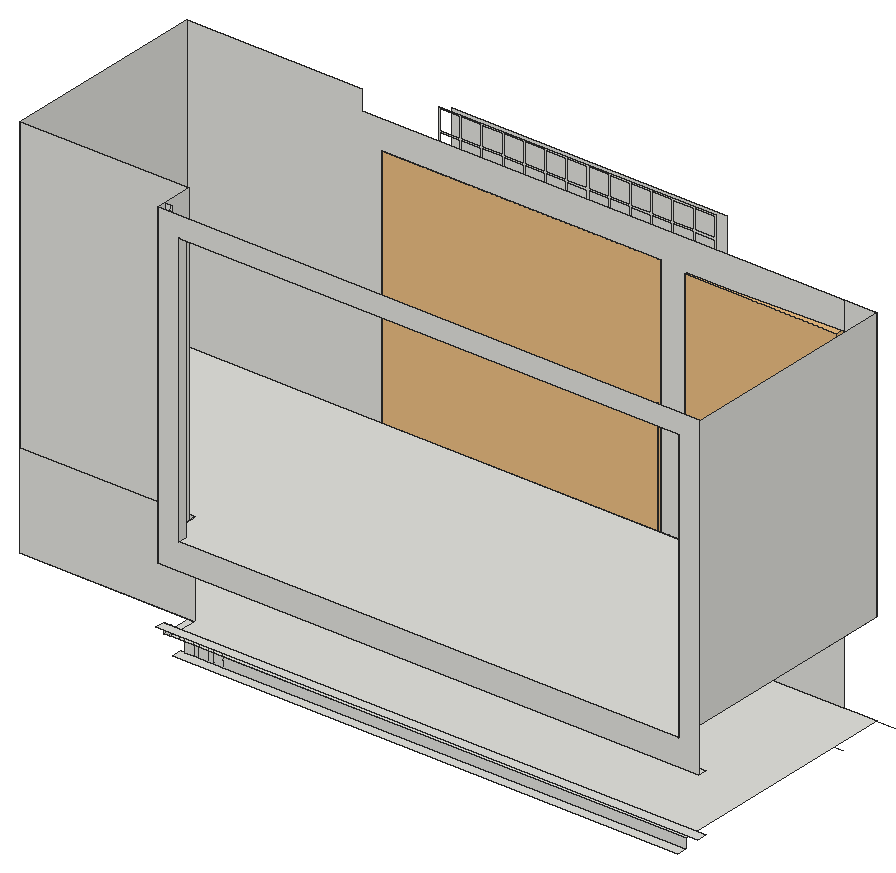
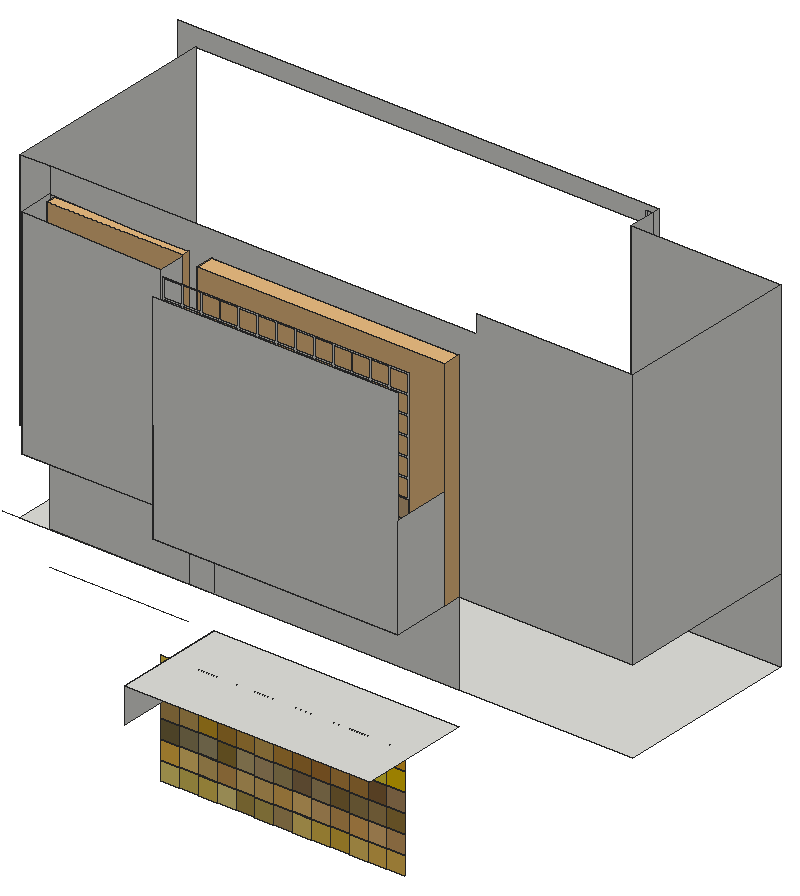
# SketchUp Ruby script. Lengths in inches.
U = 1.inch
M = Sketchup.active_model
def pt(a) = Geom::Point3d.new(a.map { |v| v * U })
def face(e, loops, mat)
  f = e.add_face(loops[0].map { |a| pt(a) })
  loops[1..].each { |l| e.add_face(l.map { |a| pt(a) }).erase! }
  f.material = f.back_material = mat if mat
  f
end
# faces: each face lists its corners as indices into pts; further lists are holes
def faces(e, pts, list, mat = nil) = list.each { |f| face(e, (f[0].is_a?(Array) ? f : [f]).map { |l| l.map { |i| pts[i] } }, mat) }
# xy, xz, yz: faces in a plane at the given z, y or x. An outline is a flat list of corners, or four numbers for a rectangle; further outlines are holes
def ring(l) = l.size == 4 ? [[l[0], l[1]], [l[2], l[1]], [l[2], l[3]], [l[0], l[3]]] : l.each_slice(2).to_a
def flat(e, list, mat, &to3) = list.each { |f| face(e, (f[0].is_a?(Array) ? f : [f]).map { |l| ring(l).map { |u, v| to3.(u, v) } }, mat) }
def xy(e, z, list, mat = nil) = flat(e, list, mat) { |x, y| [x, y, z] }
def xz(e, y, list, mat = nil) = flat(e, list, mat) { |x, z| [x, y, z] }
def yz(e, x, list, mat = nil) = flat(e, list, mat) { |y, z| [x, y, z] }
def lines(e, pts, list) = list.each { |a, b| e.add_line(pt(pts[a]), pt(pts[b])) }
# prism: a flat outline (further loops are holes) pulled along v
def prism(e, loops, v, mat = nil)
  f = face(e, loops, mat); d = Geom::Vector3d.new(v.map { |x| x * U })
  f.pushpull(f.normal.samedirection?(d) ? d.length : -d.length)
end
def box(e, o, s, mat = nil) = prism(e, [[o, [o[0] + s[0], o[1], o[2]], [o[0] + s[0], o[1] + s[1], o[2]], [o[0], o[1] + s[1], o[2]]]], [0, 0, s[2]], mat)
def at(x, y, z, deg = 0) = Geom::Transformation.translation(pt([x, y, z])) * Geom::Transformation.rotation(ORIGIN, Z_AXIS, deg.degrees)
def axes(o, x, y, z) = Geom::Transformation.new([*x, 0, *y, 0, *z, 0, *pt(o).to_a, 1])
def part(name) = M.definitions.add(name)
# library, detail: a bought-in or finely detailed component or shape, given as its bounding box
def library(name, o, s) = part(name).tap { |d| box(d.entities, o, s) }
def detail(e, o, s) = box(e.add_group.entities, o, s)
def put(e, d, t, mat = nil) = e.add_instance(d, t).tap { |i| i.material = mat if mat }
def group(e, t, mat = nil) = e.add_group.tap { |g| g.transformation = t; g.material = mat if mat }.entities
root = M.entities
M.materials.add("SW 0012 Empire Gold").color = [192, 162, 108]
M.materials.add("SW 0028 Caen Stone").color = [234, 212, 175]
M.materials.add("SW 0030 Colonial Yellow").color = [235, 202, 133]
M.materials.add("SW 0043 Peristyle Brass").color = [171, 151, 98]
M.materials.add("SW 0044 Hubbard Squash").color = [228, 196, 137]
M.materials.add("SW 0067 Belvedere Cream").color = [236, 208, 158]
M.materials.add("SW 0078 Sunbeam Yellow").color = [236, 216, 155]
M.materials.add("SW 2813 Downing Straw").color = [196, 173, 119]
M.materials.add("SW 2814 Rookwood Antique Gold").color = [158, 131, 78]
M.materials.add("SW 2817 Rookwood Amber").color = [185, 135, 62]
M.materials.add("SW 2831 Classical Gold").color = [230, 191, 112]
M.materials.add("SW 2834 Birdseye Maple").color = [221, 199, 142]
M.materials.add("SW 2853 New Colonial Yellow").color = [211, 178, 125]
M.materials.add("SW 2857 Peace Yellow").color = [231, 210, 153]
M.materials.add("SW 2858 Harvest Gold").color = [215, 167, 103]
M.materials.add("SW 2865 Classical Yellow").color = [244, 218, 144]
M.materials.add("SW 6113 Interactive Cream").color = [226, 206, 173]
M.materials.add("SW 6114 Bagel").color = [213, 185, 146]
M.materials.add("SW 6115 Totally Tan").color = [202, 170, 129]
M.materials.add("SW 6116 Tatami Tan").color = [184, 148, 100]
M.materials.add("SW 6117 Smokey Topaz").color = [164, 127, 83]
M.materials.add("SW 6118 Leather Bound").color = [139, 102, 57]
M.materials.add("SW 6120 Believable Buff").color = [216, 202, 167]
M.materials.add("SW 6121 Whole Wheat").color = [203, 185, 145]
M.materials.add("SW 6122 Camelback").color = [194, 175, 133]
M.materials.add("SW 6123 Baguette").color = [175, 151, 103]
M.materials.add("SW 6127 Ivoire").color = [224, 209, 170]
M.materials.add("SW 6128 Blonde").color = [217, 193, 145]
M.materials.add("SW 6129 Restrained Gold").color = [206, 183, 131]
M.materials.add("SW 6130 Mannered Gold").color = [189, 159, 99]
M.materials.add("SW 6131 Chamois").color = [172, 141, 84]
M.materials.add("SW 6132 Relic Bronze").color = [143, 113, 59]
M.materials.add("SW 6134 Netsuke").color = [220, 210, 175]
M.materials.add("SW 6135 Ecru").color = [206, 193, 149]
M.materials.add("SW 6136 Harmonic Tan").color = [194, 179, 136]
M.materials.add("SW 6137 Burlap").color = [170, 155, 114]
M.materials.add("SW 6138 Artifact").color = [151, 136, 95]
M.materials.add("SW 6139 Mossy Gold").color = [124, 107, 64]
M.materials.add("SW 6365 Cachet Cream").color = [240, 220, 183]
M.materials.add("SW 6366 Ambitious Amber").color = [238, 208, 148]
M.materials.add("SW 6367 Viva Gold").color = [227, 182, 114]
M.materials.add("SW 6368 Bakelite Gold").color = [212, 162, 89]
M.materials.add("SW 6369 Tassel").color = [195, 143, 67]
M.materials.add("SW 6370 Saucy Gold").color = [179, 122, 51]
M.materials.add("SW 6372 Inviting Ivory").color = [239, 218, 175]
M.materials.add("SW 6373 Harvester").color = [232, 201, 137]
M.materials.add("SW 6374 Torchlight").color = [226, 185, 106]
M.materials.add("SW 6375 Honeycomb").color = [210, 161, 84]
M.materials.add("SW 6376 Gold Coast").color = [195, 143, 57]
M.materials.add("SW 6377 Butterscotch").color = [180, 128, 52]
M.materials.add("SW 6379 Jersey Cream").color = [239, 224, 185]
M.materials.add("SW 6380 Humble Gold").color = [232, 206, 147]
M.materials.add("SW 6381 Anjou Pear").color = [217, 181, 105]
M.materials.add("SW 6382 Ceremonial Gold").color = [208, 167, 85]
M.materials.add("SW 6383 Golden Rule").color = [199, 153, 65]
M.materials.add("SW 6384 Cut The Mustard").color = [182, 135, 47]
M.materials.add("SW 6387 Compatible Cream").color = [229, 206, 156]
M.materials.add("SW 6388 Golden Fleece").color = [227, 182, 114]
M.materials.add("SW 6389 Butternut").color = [200, 164, 90]
M.materials.add("SW 6390 Bosc Pear").color = [188, 151, 83]
M.materials.add("SW 6391 Gallant Gold").color = [161, 128, 61]
M.materials.add("SW 6393 Convivial Yellow").color = [229, 218, 173]
M.materials.add("SW 6394 Sequin").color = [220, 200, 139]
M.materials.add("SW 6395 Alchemy").color = [197, 171, 86]
M.materials.add("SW 6396 Different Gold").color = [183, 156, 75]
M.materials.add("SW 6397 Nankeen").color = [162, 135, 46]
M.materials.add("SW 6398 Sconce Gold").color = [151, 121, 51]
M.materials.add("SW 6400 Lucent Yellow").color = [223, 213, 164]
M.materials.add("SW 6407 Ancestral Gold").color = [218, 210, 164]
M.materials.add("SW 6659 Captivating Cream").color = [243, 220, 176]
M.materials.add("SW 6660 Honey Blush").color = [243, 211, 152]
M.materials.add("SW 6661 Papaya").color = [238, 189, 120]
M.materials.add("SW 6662 Summer Day").color = [234, 176, 94]
M.materials.add("SW 6663 Saffron Thread").color = [223, 158, 74]
M.materials.add("SW 6666 Enjoyable Yellow").color = [244, 218, 167]
M.materials.add("SW 6667 Afterglow").color = [243, 209, 138]
M.materials.add("SW 6668 Sunrise").color = [242, 197, 116]
M.materials.add("SW 6669 Yarrow").color = [231, 180, 89]
M.materials.add("SW 6670 Gold Crest").color = [221, 159, 46]
M.materials.add("SW 6671 Curry").color = [214, 148, 38]
M.materials.add("SW 6673 Banana Cream").color = [243, 226, 174]
M.materials.add("SW 6674 Jonquil").color = [244, 216, 142]
M.materials.add("SW 6675 Afternoon").color = [248, 209, 116]
M.materials.add("SW 6676 Butterfield").color = [244, 196, 86]
M.materials.add("SW 6677 Goldenrod").color = [244, 196, 86]
M.materials.add("SW 6678 Sunflower").color = [223, 162, 35]
M.materials.add("SW 6680 Friendly Yellow").color = [241, 228, 176]
M.materials.add("SW 6681 Butter Up").color = [243, 225, 159]
M.materials.add("SW 6682 June Day").color = [242, 210, 111]
M.materials.add("SW 6683 Bee").color = [235, 196, 79]
M.materials.add("SW 6684 Brittlebush").color = [228, 184, 61]
M.materials.add("SW 6685 Trinket").color = [209, 161, 37]
M.materials.add("SW 6687 Lantern Light").color = [241, 228, 173]
M.materials.add("SW 6688 Solaria").color = [242, 221, 140]
M.materials.add("SW 6689 Overjoy").color = [233, 203, 89]
M.materials.add("SW 6690 Gambol Gold").color = [220, 186, 63]
M.materials.add("SW 6691 Glitzy Gold").color = [208, 168, 18]
M.materials.add("SW 6692 Auric").color = [191, 145, 0]
M.materials.add("SW 6694 Glad Yellow").color = [240, 230, 169]
M.materials.add("SW 6695 Midday").color = [242, 222, 135]
M.materials.add("SW 6696 Quilt Gold").color = [227, 203, 95]
M.materials.add("SW 6697 Nugget").color = [211, 184, 67]
M.materials.add("SW 6698 Kingdom Gold").color = [202, 173, 37]
M.materials.add("SW 6699 Crispy Gold").color = [191, 161, 37]
M.materials.add("SW 6701 Moonraker").color = [234, 231, 176]
M.materials.add("SW 6888 Pizazz Peach").color = [243, 202, 146]
M.materials.add("SW 6889 Stirring Orange").color = [243, 181, 96]
M.materials.add("SW 6890 Osage Orange").color = [243, 166, 60]
M.materials.add("SW 6894 Forceful Orange").color = [242, 160, 0]
M.materials.add("SW 6895 Laughing Orange").color = [242, 160, 0]
M.materials.add("SW 6896 Solé").color = [243, 226, 157]
M.materials.add("SW 6897 Sundance").color = [245, 206, 103]
M.materials.add("SW 6898 Social Butterfly").color = [247, 193, 71]
M.materials.add("SW 6899 Nasturtiumb").color = [246, 178, 33]
M.materials.add("SW 6900 Optimistic Yellow").color = [242, 228, 163]
M.materials.add("SW 6901 Daffodil").color = [246, 223, 119]
M.materials.add("SW 6902 Decisive Yellow").color = [248, 211, 68]
M.materials.add("SW 6903 Cheerful").color = [250, 208, 0]
M.materials.add("SW 6904 Gusto Gold").color = [245, 181, 0]
M.materials.add("SW 6905 Goldfinch").color = [249, 192, 0]
M.materials.add("SW 6906 Citrus").color = [251, 205, 0]
M.materials.add("SW 6907 Forsythia").color = [251, 210, 0]
M.materials.add("SW 6908 Fun Yellow").color = [242, 235, 145]
M.materials.add("SW 6909 Lemon Twist").color = [248, 227, 86]
M.materials.add("SW 6910 Daisy").color = [246, 220, 49]
M.materials.add("SW 6911 Confident Yellow").color = [245, 214, 0]
M.materials.add("SW 6912 Glisten Yellow").color = [240, 235, 169]
M.materials.add("SW 7537 Irish Cream").color = [227, 211, 186]
M.materials.add("SW 7676 Paper Lantern").color = [240, 224, 198]
M.materials.add("SW 7677 Gold Vessel").color = [233, 187, 138]
M.materials.add("SW 7678 Cottage Cream").color = [236, 219, 189]
M.materials.add("SW 7679 Golden Gate").color = [217, 176, 132]
M.materials.add("SW 7680 Lanyard").color = [191, 153, 116]
M.materials.add("SW 7681 Tea Light").color = [246, 227, 194]
M.materials.add("SW 7682 Bee_s Wax").color = [233, 192, 136]
M.materials.add("SW 7683 Buff").color = [242, 225, 197]
M.materials.add("SW 7684 Concord Buff").color = [239, 216, 182]
M.materials.add("SW 7685 White Raisin").color = [228, 192, 140]
M.materials.add("SW 7686 Hinoki").color = [246, 220, 183]
M.materials.add("SW 7687 August Moon").color = [231, 199, 161]
M.materials.add("SW 7688 Sundew").color = [223, 206, 176]
M.materials.add("SW 7689 Row House Tan").color = [211, 187, 159]
M.materials.add("SW 7690 Townhall Tan").color = [194, 171, 140]
M.materials.add("SW 7691 Biltmore Buff").color = [225, 202, 161]
M.materials.add("SW 7692 Cupola Yellow").color = [219, 188, 144]
M.materials.add("SW 7693 Stonebriar").color = [203, 172, 128]
M.materials.add("SW 7694 Dromedary Camel").color = [203, 175, 136]
M.materials.add("SW 7695 Mesa Tan").color = [190, 160, 124]
M.materials.add("SW 7696 Toasted Pine Nut").color = [218, 199, 167]
M.materials.add("SW 7697 Safari").color = [203, 179, 141]
M.materials.add("SW 7698 Straw Harvest").color = [217, 199, 161]
M.materials.add("SW 7699 Rustic City").color = [188, 160, 113]
M.materials.add("SW 7700 Olde World Gold").color = [145, 116, 76]
M.materials.add("SW 7717 Ligonier Tan").color = [211, 178, 143]
c1 = library("Group6\#1",[-22.44,-5.97,0],[42.52,9.29,84.25])
c2 = library("Glass_door",[70.54,1.5625,0],[78.74,7.87,82.68])
xy(root,793.31,[[1349.53,376.08,1604.22,492.39]])
xy(root,818.54,[[1339.44,147.16,1805.83,155.91]])
xy(root,827.6,[[1330.44,155.91,1330.44,183.72,1169.07,183.72,1169.07,376.08,1805.83,376.08,1805.83,155.91],[1324.51,155.91,1330.44,183.72]])
xy(root,836.67,[[1323.88,147.16,1824.45,155.91]])
xy(root,889.6875,[[1324.51,147.66,1824.45,155.91]])
xy(root,900.37,[[1324.51,155.91,1330.44,183.72]])
xy(root,914.18,[[1344.39,147.66,1805.83,147.66,1805.83,376.08,1169.07,376.08,1169.07,183.72,1330.44,183.72,1330.44,155.91,1344.39,155.91],[1349.53,376.08,1604.22,455.83],[1630.81,376.08,1775.37,412.2]])
xz(root,147.66,[[[1324.51,889.6875,1824.45,1184.06],[1344.39,914.18,1805.83,1165.72]]])
xz(root,155.91,[[1342.94,818.54,1351.36,827.6],[1351.36,818.54,1356.32,827.6],[1356.32,818.54,1364.74,827.6],[1364.74,818.54,1369.69,827.6],[1369.69,818.54,1378.11,827.6],
  [1378.11,818.54,1805.83,827.6],[1323.88,827.6,1324.61,836.67],[1324.61,827.6,1329.57,836.67],[1329.57,827.6,1330.44,836.67],[1324.51,889.6875,1324.61,900.37],
  [1324.61,889.6875,1329.57,900.37],[1329.57,889.6875,1330.44,900.37],[1324.51,900.37,1324.61,1184.06],[1324.61,900.37,1329.57,1184.06],[1329.57,900.37,1329.57,1184.06,1330.95,1184.06,1330.95,1165.72,1337.99,1165.72,1337.99,914.18,1330.44,914.18,1330.44,900.37],
  [1337.99,914.18,1342.94,1165.72],[1342.94,914.18,1344.39,1165.72]])
xz(root,183.72,[[1169.07,827.6,1330.44,827.6,1330.44,900.37,1324.51,900.37,1324.51,914.18,1169.07,914.18],[1324.51,900.37,1330.44,914.18],[1169.07,914.18,1324.51,1184.06]])
xz(root,376.08,[[1349.53,827.6,1604.22,914.18],[1604.22,827.6,1630.81,914.18],[1630.81,827.6,1775.37,914.18],[1169.07,914.18,1349.53,914.18,1349.53,1139.55,1604.22,1139.55,1604.22,914.18,1630.81,914.18,1630.81,1136.29,1775.37,1139.55,1775.37,1165.72,1330.95,1165.72,1330.95,1184.06,1169.07,1184.06],[1775.37,914.18,1805.83,1165.72]])
xz(root,412.2,[[1630.81,914.18,1775.37,914.18,1775.37,1139.55,1630.81,1136.29]])
xz(root,434.23,[[1476.59,715.37,1495.24,734.02]],"SW 0043 Peristyle Brass")
xz(root,434.23,[[1515.79,715.37,1534.44,734.02]],"SW 2813 Downing Straw")
xz(root,434.23,[[1398.18,715.37,1416.83,734.02]],"SW 2814 Rookwood Antique Gold")
xz(root,434.23,[[1398.18,734.97,1416.83,753.625]],"SW 2817 Rookwood Amber")
xz(root,434.23,[[1515.79,695.77,1534.44,714.42]],"SW 2831 Classical Gold")
xz(root,434.23,[[1358.98,695.77,1377.63,714.42]],"SW 2858 Harvest Gold")
xz(root,434.23,[[1358.98,734.97,1377.63,753.625]],"SW 6116 Tatami Tan")
xz(root,434.23,[[1594.2,754.58,1612.85,773.23]],"SW 6117 Smokey Topaz")
xz(root,434.23,[[1378.58,734.97,1397.23,753.625]],"SW 6118 Leather Bound")
xz(root,434.23,[[1437.38,715.37,1456.04,734.02]],"SW 6123 Baguette")
xz(root,434.23,[[1476.59,676.17,1495.24,694.82]],"SW 6130 Mannered Gold")
xz(root,434.23,[[1378.58,715.37,1397.23,734.02]],"SW 6131 Chamois")
xz(root,434.23,[[1417.78,715.37,1436.43,734.02]],"SW 6132 Relic Bronze")
xz(root,434.23,[[1555,715.37,1573.65,734.02]],"SW 6137 Burlap")
xz(root,434.23,[[1574.6,715.37,1593.25,734.02]],"SW 6138 Artifact")
xz(root,434.23,[[1594.2,715.37,1612.85,734.02]],"SW 6139 Mossy Gold")
xz(root,434.23,[[1437.38,695.77,1456.04,714.42]],"SW 6367 Viva Gold")
xz(root,434.23,[[1417.78,695.77,1436.43,714.42]],"SW 6368 Bakelite Gold")
xz(root,434.23,[[1417.78,734.97,1436.43,753.625]],"SW 6369 Tassel")
xz(root,434.23,[[1437.38,734.97,1456.04,753.625]],"SW 6370 Saucy Gold")
xz(root,434.23,[[1496.19,695.77,1514.84,714.42]],"SW 6374 Torchlight")
xz(root,434.23,[[1535.39,695.77,1554.05,714.42]],"SW 6375 Honeycomb")
xz(root,434.23,[[1476.59,734.97,1495.24,753.625]],"SW 6376 Gold Coast")
xz(root,434.23,[[1456.99,734.97,1475.64,753.625]],"SW 6377 Butterscotch")
xz(root,434.23,[[1555,695.77,1573.65,714.42]],"SW 6381 Anjou Pear")
xz(root,434.23,[[1496.19,734.97,1514.84,753.625]],"SW 6382 Ceremonial Gold")
xz(root,434.23,[[1515.79,734.97,1534.44,753.625]],"SW 6383 Golden Rule")
xz(root,434.23,[[1535.39,734.97,1554.05,753.625]],"SW 6384 Cut The Mustard")
xz(root,434.23,[[1574.6,734.97,1593.25,753.625]],"SW 6389 Butternut")
xz(root,434.23,[[1594.2,734.97,1612.85,753.625]],"SW 6390 Bosc Pear")
xz(root,434.23,[[1358.98,715.37,1377.63,734.02]],"SW 6391 Gallant Gold")
xz(root,434.23,[[1496.19,676.17,1514.84,694.82]],"SW 6395 Alchemy")
xz(root,434.23,[[1515.79,676.17,1534.44,694.82]],"SW 6396 Different Gold")
xz(root,434.23,[[1574.6,754.58,1593.25,773.23]],"SW 6397 Nankeen")
xz(root,434.23,[[1535.39,715.37,1554.05,734.02]],"SW 6398 Sconce Gold")
xz(root,434.23,[[1378.58,695.77,1397.23,714.42]],"SW 6661 Papaya")
xz(root,434.23,[[1398.18,695.77,1416.83,714.42]],"SW 6662 Summer Day")
xz(root,434.23,[[1456.99,774.18,1475.64,792.83]],"SW 6663 Saffron Thread")
xz(root,434.23,[[1456.99,695.77,1475.64,714.42]],"SW 6668 Sunrise")
xz(root,434.23,[[1476.59,695.77,1495.24,714.42]],"SW 6669 Yarrow")
xz(root,434.23,[[1496.19,774.18,1514.84,792.83]],"SW 6670 Gold Crest")
xz(root,434.23,[[1476.59,774.18,1495.24,792.83]],"SW 6671 Curry")
xz(root,434.23,[[1574.6,695.77,1593.25,714.42]],"SW 6675 Afternoon")
xz(root,434.23,[[1358.98,676.17,1377.63,694.82]],"SW 6676 Butterfield")
xz(root,434.23,[[1378.58,676.17,1397.23,694.82]],"SW 6677 Goldenrod")
xz(root,434.23,[[1515.79,774.18,1534.44,792.83]],"SW 6678 Sunflower")
xz(root,434.23,[[1456.99,676.17,1475.64,694.82]],"SW 6682 June Day")
xz(root,434.23,[[1437.38,676.17,1456.04,694.82]],"SW 6683 Bee")
xz(root,434.23,[[1417.78,676.17,1436.43,694.82]],"SW 6684 Brittlebush")
xz(root,434.23,[[1555,734.97,1573.65,753.625]],"SW 6685 Trinket")
xz(root,434.23,[[1555,676.17,1573.65,694.82]],"SW 6689 Overjoy")
xz(root,434.23,[[1456.99,754.58,1475.64,773.23]],"SW 6690 Gambol Gold")
xz(root,434.23,[[1476.59,754.58,1495.24,773.23]],"SW 6691 Glitzy Gold")
xz(root,434.23,[[1496.19,754.58,1514.84,773.23]],"SW 6692 Auric")
xz(root,434.23,[[1535.39,676.17,1554.05,694.82]],"SW 6695 Midday")
xz(root,434.23,[[1574.6,676.17,1593.25,694.82]],"SW 6696 Quilt Gold")
xz(root,434.23,[[1515.79,754.58,1534.44,773.23]],"SW 6697 Nugget")
xz(root,434.23,[[1535.39,754.58,1554.05,773.23]],"SW 6698 Kingdom Gold")
xz(root,434.23,[[1555,754.58,1573.65,773.23]],"SW 6699 Crispy Gold")
xz(root,434.23,[[1437.38,774.18,1456.04,792.83]],"SW 6889 Stirring Orange")
xz(root,434.23,[[1417.78,774.18,1436.43,792.83]],"SW 6890 Osage Orange")
xz(root,434.23,[[1398.18,774.18,1416.83,792.83]],"SW 6894 Forceful Orange")
xz(root,434.23,[[1378.58,774.18,1397.23,792.83]],"SW 6895 Laughing Orange")
xz(root,434.23,[[1398.18,676.17,1416.83,694.82]],"SW 6897 Sundance")
xz(root,434.23,[[1594.2,695.77,1612.85,714.42]],"SW 6898 Social Butterfly")
xz(root,434.23,[[1358.98,774.18,1377.63,792.83]],"SW 6899 Nasturtiumb")
xz(root,434.23,[[1594.2,676.17,1612.85,694.82]],"SW 6901 Daffodil")
xz(root,434.23,[[1594.2,774.18,1612.85,792.83]],"SW 6902 Decisive Yellow")
xz(root,434.23,[[1574.6,774.18,1593.25,792.83]],"SW 6903 Cheerful")
xz(root,434.23,[[1535.39,774.18,1554.05,792.83]],"SW 6904 Gusto Gold")
xz(root,434.23,[[1555,774.18,1573.65,792.83]],"SW 6905 Goldfinch")
xz(root,434.23,[[1358.98,754.58,1377.63,773.23]],"SW 6906 Citrus")
xz(root,434.23,[[1398.18,754.58,1416.83,773.23]],"SW 6907 Forsythia")
xz(root,434.23,[[1417.78,754.58,1436.43,773.23]],"SW 6909 Lemon Twist")
xz(root,434.23,[[1378.58,754.58,1397.23,773.23]],"SW 6910 Daisy")
xz(root,434.23,[[1437.38,754.58,1456.04,773.23]],"SW 6911 Confident Yellow")
xz(root,434.23,[[1496.19,715.37,1514.84,734.02]],"SW 7699 Rustic City")
xz(root,434.23,[[1456.99,715.37,1475.64,734.02]],"SW 7700 Olde World Gold")
xz(root,438.51,[[[1351.73,913.23,1607.51,1149.41],[1587.9,1031.8,1606.56,1050.45],[1352.68,1031.8,1371.33,1050.45],[1372.28,1031.8,1390.93,1050.45],[1391.88,1031.8,1410.54,1050.45],[1411.49,1031.8,1430.14,1050.45],[1431.09,1031.8,1449.74,1050.45],[1450.69,1031.8,1469.34,1050.45],[1470.29,1031.8,1488.94,1050.45],[1489.89,1031.8,1508.55,1050.45],[1509.5,1031.8,1528.15,1050.45],[1529.1,1031.8,1547.75,1050.45],[1548.7,1031.8,1567.35,1050.45],[1568.3,1031.8,1586.95,1050.45],[1587.9,1012.19,1606.56,1030.85],[1352.68,1012.19,1371.33,1030.85],[1372.28,1012.19,1390.93,1030.85],[1391.88,1012.19,1410.54,1030.85],[1411.49,1012.19,1430.14,1030.85],[1431.09,1012.19,1449.74,1030.85],[1450.69,1012.19,1469.34,1030.85],[1470.29,1012.19,1488.94,1030.85],[1489.89,1012.19,1508.55,1030.85],[1509.5,1012.19,1528.15,1030.85],[1529.1,1012.19,1547.75,1030.85],[1548.7,1012.19,1567.35,1030.85],[1568.3,1012.19,1586.95,1030.85],[1587.9,992.59,1606.56,1011.24],[1587.9,1051.4,1606.56,1070.05],[1587.9,1071,1606.56,1089.65],[1587.9,1090.6,1606.56,1109.25],[1587.9,1110.2,1606.56,1128.86],[1587.9,914.18,1606.56,932.84],[1587.9,953.39,1606.56,972.04],[1352.68,1110.2,1371.33,1128.86],[1352.68,1090.6,1371.33,1109.25],[1352.68,1071,1371.33,1089.65],[1352.68,1051.4,1371.33,1070.05],[1352.68,992.59,1371.33,1011.24],[1372.28,1110.2,1390.93,1128.86],[1372.28,1090.6,1390.93,1109.25],[1372.28,1071,1390.93,1089.65],[1372.28,1051.4,1390.93,1070.05],[1372.28,992.59,1390.93,1011.24],[1391.88,992.59,1410.54,1011.24],[1391.88,1051.4,1410.54,1070.05],[1391.88,1071,1410.54,1089.65],[1391.88,1090.6,1410.54,1109.25],[1391.88,1110.2,1410.54,1128.86],[1411.49,992.59,1430.14,1011.24],[1411.49,1051.4,1430.14,1070.05],[1411.49,1071,1430.14,1089.65],[1411.49,1090.6,1430.14,1109.25],[1411.49,1110.2,1430.14,1128.86],[1587.9,933.79,1606.56,952.4375],[1352.68,914.18,1371.33,932.84],[1372.28,914.18,1390.93,932.84],[1391.88,914.18,1410.54,932.84],[1411.49,914.18,1430.14,932.84],[1431.09,1051.4,1449.74,1070.05],[1431.09,992.59,1449.74,1011.24],[1431.09,1090.6,1449.74,1109.25],[1431.09,1110.2,1449.74,1128.86],[1431.09,1071,1449.74,1089.65],[1450.69,1110.2,1469.34,1128.86],[1450.69,1090.6,1469.34,1109.25],[1450.69,1071,1469.34,1089.65],[1450.69,1051.4,1469.34,1070.05],[1450.69,992.59,1469.34,1011.24],[1470.29,1110.2,1488.94,1128.86],[1470.29,1090.6,1488.94,1109.25],[1470.29,992.59,1488.94,1011.24],[1470.29,1051.4,1488.94,1070.05],[1470.29,1071,1488.94,1089.65],[1489.89,992.59,1508.55,1011.24],[1489.89,1051.4,1508.55,1070.05],[1489.89,1071,1508.55,1089.65],[1489.89,1090.6,1508.55,1109.25],[1489.89,1110.2,1508.55,1128.86],[1509.5,992.59,1528.15,1011.24],[1509.5,1051.4,1528.15,1070.05],[1509.5,1071,1528.15,1089.65],[1509.5,1090.6,1528.15,1109.25],[1509.5,1110.2,1528.15,1128.86],[1529.1,992.59,1547.75,1011.24],[1529.1,1051.4,1547.75,1070.05],[1529.1,1071,1547.75,1089.65],[1529.1,1090.6,1547.75,1109.25],[1529.1,1110.2,1547.75,1128.86],[1548.7,992.59,1567.35,1011.24],[1548.7,1051.4,1567.35,1070.05],[1548.7,1071,1567.35,1089.65],[1548.7,1090.6,1567.35,1109.25],[1548.7,1110.2,1567.35,1128.86],[1568.3,992.59,1586.95,1011.24],[1568.3,1051.4,1586.95,1070.05],[1568.3,1071,1586.95,1089.65],[1568.3,1090.6,1586.95,1109.25],[1568.3,1110.2,1586.95,1128.86],[1352.68,953.39,1371.33,972.04],[1372.28,953.39,1390.93,972.04],[1391.88,953.39,1410.54,972.04],[1411.49,953.39,1430.14,972.04],[1431.09,914.18,1449.74,932.84],[1450.69,914.18,1469.34,932.84],[1470.29,914.18,1488.94,932.84],[1489.89,914.18,1508.55,932.84],[1509.5,914.18,1528.15,932.84],[1529.1,914.18,1547.75,932.84],[1548.7,914.18,1567.35,932.84],[1568.3,914.18,1586.95,932.84],[1352.68,933.79,1371.33,952.4375],[1372.28,933.79,1390.93,952.4375],[1391.88,933.79,1410.54,952.4375],[1411.49,933.79,1430.14,952.4375],[1431.09,953.39,1449.74,972.04],[1450.69,953.39,1469.34,972.04],[1470.29,953.39,1488.94,972.04],[1489.89,953.39,1508.55,972.04],[1509.5,953.39,1528.15,972.04],[1529.1,953.39,1547.75,972.04],[1548.7,953.39,1567.35,972.04],[1568.3,953.39,1586.95,972.04],[1431.09,933.79,1449.74,952.4375],[1450.69,933.79,1469.34,952.4375],[1470.29,933.79,1488.94,952.4375],[1489.89,933.79,1508.55,952.4375],[1509.5,933.79,1528.15,952.4375],[1529.1,933.79,1547.75,952.4375],[1548.7,933.79,1567.35,952.4375],[1568.3,933.79,1586.95,952.4375],[1587.9,1129.81,1606.56,1148.46],[1587.9,972.99,1606.56,991.64],[1352.68,1129.81,1371.33,1148.46],[1352.68,972.99,1371.33,991.64],[1372.28,972.99,1390.93,991.64],[1372.28,1129.81,1390.93,1148.46],[1391.88,1129.81,1410.54,1148.46],[1391.88,972.99,1410.54,991.64],[1411.49,1129.81,1430.14,1148.46],[1411.49,972.99,1430.14,991.64],[1431.09,972.99,1449.74,991.64],[1431.09,1129.81,1449.74,1148.46],[1450.69,972.99,1469.34,991.64],[1450.69,1129.81,1469.34,1148.46],[1470.29,1129.81,1488.94,1148.46],[1470.29,972.99,1488.94,991.64],[1489.89,1129.81,1508.55,1148.46],[1489.89,972.99,1508.55,991.64],[1509.5,1129.81,1528.15,1148.46],[1509.5,972.99,1528.15,991.64],[1529.1,1129.81,1547.75,1148.46],[1529.1,972.99,1547.75,991.64],[1548.7,1129.81,1567.35,1148.46],[1548.7,972.99,1567.35,991.64],[1568.3,1129.81,1586.95,1148.46],[1568.3,972.99,1586.95,991.64]],[1568.3,914.18,1586.95,932.84],[1587.9,914.18,1606.56,932.84]])
xz(root,438.51,[[1470.29,1012.19,1488.94,1030.85]],"SW 0012 Empire Gold")
xz(root,438.51,[[1372.28,933.79,1390.93,952.4375]],"SW 0028 Caen Stone")
xz(root,438.51,[[1352.68,953.39,1371.33,972.04]],"SW 0030 Colonial Yellow")
xz(root,438.51,[[1489.89,972.99,1508.55,991.64]],"SW 0044 Hubbard Squash")
xz(root,438.51,[[1450.69,972.99,1469.34,991.64]],"SW 0067 Belvedere Cream")
xz(root,438.51,[[1431.09,992.59,1449.74,1011.24]],"SW 0078 Sunbeam Yellow")
xz(root,438.51,[[1568.3,1012.19,1586.95,1030.85]],"SW 2834 Birdseye Maple")
xz(root,438.51,[[1352.68,972.99,1371.33,991.64]],"SW 2853 New Colonial Yellow")
xz(root,438.51,[[1548.7,972.99,1567.35,991.64]],"SW 2857 Peace Yellow")
xz(root,438.51,[[1450.69,953.39,1469.34,972.04]],"SW 2865 Classical Yellow")
xz(root,438.51,[[1411.49,933.79,1430.14,952.4375]],"SW 6113 Interactive Cream")
xz(root,438.51,[[1372.28,1012.19,1390.93,1030.85]],"SW 6114 Bagel")
xz(root,438.51,[[1352.68,1012.19,1371.33,1030.85]],"SW 6115 Totally Tan")
xz(root,438.51,[[1450.69,914.18,1469.34,932.84]],"SW 6120 Believable Buff")
xz(root,438.51,[[1450.69,992.59,1469.34,1011.24]],"SW 6121 Whole Wheat")
xz(root,438.51,[[1470.29,992.59,1488.94,1011.24]],"SW 6122 Camelback")
xz(root,438.51,[[1411.49,914.18,1430.14,932.84]],"SW 6127 Ivoire")
xz(root,438.51,[[1352.68,992.59,1371.33,1011.24]],"SW 6128 Blonde")
xz(root,438.51,[[1372.28,992.59,1390.93,1011.24]],"SW 6129 Restrained Gold")
xz(root,438.51,[[1470.29,914.18,1488.94,932.84]],"SW 6134 Netsuke")
xz(root,438.51,[[1509.5,992.59,1528.15,1011.24]],"SW 6135 Ecru")
xz(root,438.51,[[1529.1,992.59,1547.75,1011.24]],"SW 6136 Harmonic Tan")
xz(root,438.51,[[1391.88,933.79,1410.54,952.4375]],"SW 6365 Cachet Cream")
xz(root,438.51,[[1411.49,972.99,1430.14,991.64]],"SW 6366 Ambitious Amber")
xz(root,438.51,[[1509.5,933.79,1528.15,952.4375]],"SW 6372 Inviting Ivory")
xz(root,438.51,[[1470.29,972.99,1488.94,991.64]],"SW 6373 Harvester")
xz(root,438.51,[[1568.3,933.79,1586.95,952.4375]],"SW 6379 Jersey Cream")
xz(root,438.51,[[1509.5,972.99,1528.15,991.64]],"SW 6380 Humble Gold")
xz(root,438.51,[[1352.68,914.18,1371.33,932.84]],"SW 6387 Compatible Cream")
xz(root,438.51,[[1587.9,1012.19,1606.56,1030.85]],"SW 6388 Golden Fleece")
xz(root,438.51,[[1489.89,914.18,1508.55,932.84]],"SW 6393 Convivial Yellow")
xz(root,438.51,[[1411.49,992.59,1430.14,1011.24]],"SW 6394 Sequin")
xz(root,438.51,[[1529.1,914.18,1547.75,932.84]],"SW 6400 Lucent Yellow")
xz(root,438.51,[[1548.7,914.18,1567.35,932.84]],"SW 6407 Ancestral Gold")
xz(root,438.51,[[1372.28,972.99,1390.93,991.64]],"SW 6659 Captivating Cream")
xz(root,438.51,[[1431.09,972.99,1449.74,991.64]],"SW 6660 Honey Blush")
xz(root,438.51,[[1391.88,972.99,1410.54,991.64]],"SW 6666 Enjoyable Yellow")
xz(root,438.51,[[1568.3,972.99,1586.95,991.64]],"SW 6667 Afterglow")
xz(root,438.51,[[1587.9,972.99,1606.56,991.64]],"SW 6673 Banana Cream")
xz(root,438.51,[[1372.28,953.39,1390.93,972.04]],"SW 6674 Jonquil")
xz(root,438.51,[[1391.88,953.39,1410.54,972.04]],"SW 6680 Friendly Yellow")
xz(root,438.51,[[1431.09,953.39,1449.74,972.04]],"SW 6681 Butter Up")
xz(root,438.51,[[1470.29,953.39,1488.94,972.04]],"SW 6687 Lantern Light")
xz(root,438.51,[[1529.1,953.39,1547.75,972.04]],"SW 6688 Solaria")
xz(root,438.51,[[1548.7,953.39,1567.35,972.04]],"SW 6694 Glad Yellow")
xz(root,438.51,[[1352.68,933.79,1371.33,952.4375]],"SW 6701 Moonraker")
xz(root,438.51,[[1568.3,992.59,1586.95,1011.24]],"SW 6888 Pizazz Peach")
xz(root,438.51,[[1489.89,953.39,1508.55,972.04]],"SW 6896 Solé")
xz(root,438.51,[[1509.5,953.39,1528.15,972.04]],"SW 6900 Optimistic Yellow")
xz(root,438.51,[[1568.3,953.39,1586.95,972.04]],"SW 6908 Fun Yellow")
xz(root,438.51,[[1587.9,953.39,1606.56,972.04]],"SW 6912 Glisten Yellow")
xz(root,438.51,[[1431.09,933.79,1449.74,952.4375]],"SW 7537 Irish Cream")
xz(root,438.51,[[1529.1,933.79,1547.75,952.4375]],"SW 7676 Paper Lantern")
xz(root,438.51,[[1587.9,992.59,1606.56,1011.24]],"SW 7677 Gold Vessel")
xz(root,438.51,[[1391.88,914.18,1410.54,932.84]],"SW 7678 Cottage Cream")
xz(root,438.51,[[1450.69,1012.19,1469.34,1030.85]],"SW 7679 Golden Gate")
xz(root,438.51,[[1431.09,1012.19,1449.74,1030.85]],"SW 7680 Lanyard")
xz(root,438.51,[[1489.89,933.79,1508.55,952.4375]],"SW 7681 Tea Light")
xz(root,438.51,[[1529.1,972.99,1547.75,991.64]],"SW 7682 Bee_s Wax")
xz(root,438.51,[[1470.29,933.79,1488.94,952.4375]],"SW 7683 Buff")
xz(root,438.51,[[1372.28,914.18,1390.93,932.84]],"SW 7684 Concord Buff")
xz(root,438.51,[[1411.49,953.39,1430.14,972.04]],"SW 7685 White Raisin")
xz(root,438.51,[[1587.9,933.79,1606.56,952.4375]],"SW 7686 Hinoki")
xz(root,438.51,[[1548.7,933.79,1567.35,952.4375]],"SW 7687 August Moon")
xz(root,438.51,[[1450.69,933.79,1469.34,952.4375]],"SW 7688 Sundew")
xz(root,438.51,[[1391.88,1012.19,1410.54,1030.85]],"SW 7689 Row House Tan")
xz(root,438.51,[[1411.49,1012.19,1430.14,1030.85]],"SW 7690 Townhall Tan")
xz(root,438.51,[[1391.88,992.59,1410.54,1011.24]],"SW 7691 Biltmore Buff")
xz(root,438.51,[[1548.7,1012.19,1567.35,1030.85]],"SW 7692 Cupola Yellow")
xz(root,438.51,[[1529.1,1012.19,1547.75,1030.85]],"SW 7693 Stonebriar")
xz(root,438.51,[[1509.5,1012.19,1528.15,1030.85]],"SW 7694 Dromedary Camel")
xz(root,438.51,[[1489.89,1012.19,1508.55,1030.85]],"SW 7695 Mesa Tan")
xz(root,438.51,[[1431.09,914.18,1449.74,932.84]],"SW 7696 Toasted Pine Nut")
xz(root,438.51,[[1489.89,992.59,1508.55,1011.24]],"SW 7697 Safari")
xz(root,438.51,[[1509.5,914.18,1528.15,932.84]],"SW 7698 Straw Harvest")
xz(root,438.51,[[1548.7,992.59,1567.35,1011.24]],"SW 7717 Ligonier Tan")
xz(root,455.83,[[1349.53,914.18,1604.22,1139.55]])
yz(root,1169.07,[[183.72,914.18,376.08,1184.06]])
yz(root,1324.51,[[147.66,889.6875,155.91,1184.06],[155.91,900.37,183.72,1184.06]])
yz(root,1330.44,[[155.91,900.37,183.72,914.18]])
yz(root,1344.39,[[147.66,914.18,155.91,1165.72]])
yz(root,1349.53,[[376.08,914.18,455.83,1019.96]])
yz(root,1604.22,[[376.08,756.91,492.39,793.31],[376.08,914.18,455.83,1019.96]])
yz(root,1630.81,[[376.08,914.18,412.2,1018.33],[376.08,1018.33,412.2,1136.29]])
yz(root,1775.37,[[376.08,914.18,412.2,945.29],[376.08,945.29,412.2,1139.55]])
yz(root,1805.83,[[147.66,914.18,376.08,1165.72]])
p = [[1630.81,376.08,792.46],[1775.37,376.08,792.46],[1805.83,376.08,827.6],[1824.45,376.08,827.6],[1337.99,155.91,914.18],[1337.99,155.91,889.6875],
  [1337.99,155.91,836.67],[1337.99,155.91,827.6],[1342.94,155.91,889.6875],[1342.94,155.91,914.18],[1342.94,155.91,827.6],[1342.94,155.91,836.67],
  [1351.36,155.91,836.67],[1351.36,155.91,827.6],[1364.74,155.91,836.67],[1364.74,155.91,827.6],[1356.32,155.91,827.6],[1356.32,155.91,836.67],
  [1378.11,155.91,836.67],[1378.11,155.91,827.6],[1369.69,155.91,827.6],[1369.69,155.91,836.67]]
lines(root,p,[[0,1],[2,3],[4,5],[6,7],[8,9],[10,11],[12,13],[14,15],[16,17],[18,19],[20,21]])
put(root,c1,axes([1705.13,380.02,914.18],[3.3125,0,0],[0,1.0865,0],[0,0,2.65]))
put(root,c2,axes([1119.28,372.32,914.18],[3.264,0,0],[0,2.4,0],[0,0,2.72585]))
